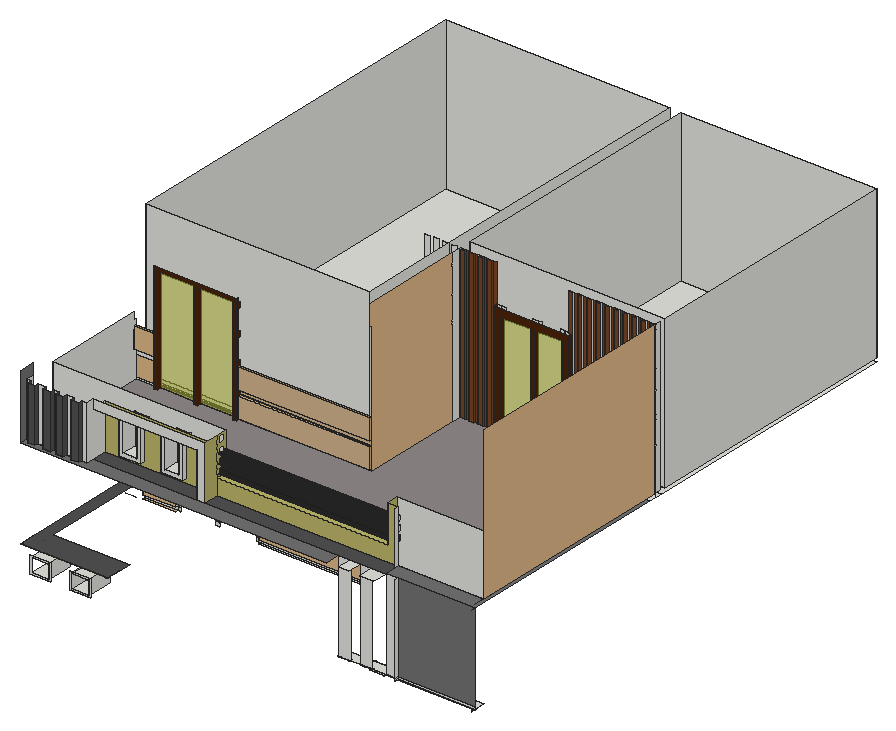
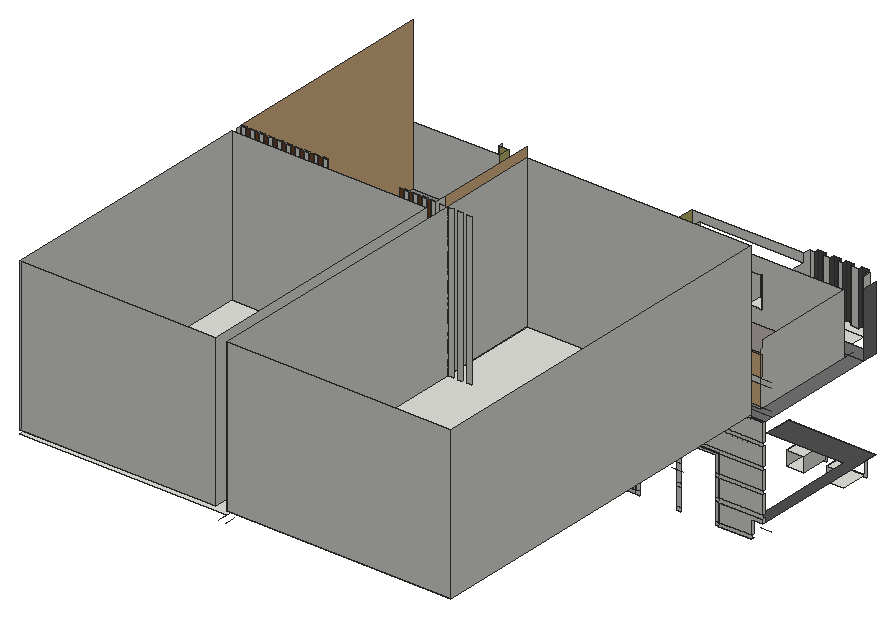
# SketchUp Ruby script. Lengths in inches.
U = 1.inch
M = Sketchup.active_model
def pt(a) = Geom::Point3d.new(a.map { |v| v * U })
def face(e, loops, mat)
  f = e.add_face(loops[0].map { |a| pt(a) })
  loops[1..].each { |l| e.add_face(l.map { |a| pt(a) }).erase! }
  f.material = f.back_material = mat if mat
  f
end
# faces: each face lists its corners as indices into pts; further lists are holes
def faces(e, pts, list, mat = nil) = list.each { |f| face(e, (f[0].is_a?(Array) ? f : [f]).map { |l| l.map { |i| pts[i] } }, mat) }
# xy, xz, yz: faces in a plane at the given z, y or x. An outline is a flat list of corners, or four numbers for a rectangle; further outlines are holes
def ring(l) = l.size == 4 ? [[l[0], l[1]], [l[2], l[1]], [l[2], l[3]], [l[0], l[3]]] : l.each_slice(2).to_a
def flat(e, list, mat, &to3) = list.each { |f| face(e, (f[0].is_a?(Array) ? f : [f]).map { |l| ring(l).map { |u, v| to3.(u, v) } }, mat) }
def xy(e, z, list, mat = nil) = flat(e, list, mat) { |x, y| [x, y, z] }
def xz(e, y, list, mat = nil) = flat(e, list, mat) { |x, z| [x, y, z] }
def yz(e, x, list, mat = nil) = flat(e, list, mat) { |y, z| [x, y, z] }
def lines(e, pts, list) = list.each { |a, b| e.add_line(pt(pts[a]), pt(pts[b])) }
# prism: a flat outline (further loops are holes) pulled along v
def prism(e, loops, v, mat = nil)
  f = face(e, loops, mat); d = Geom::Vector3d.new(v.map { |x| x * U })
  f.pushpull(f.normal.samedirection?(d) ? d.length : -d.length)
end
def box(e, o, s, mat = nil) = prism(e, [[o, [o[0] + s[0], o[1], o[2]], [o[0] + s[0], o[1] + s[1], o[2]], [o[0], o[1] + s[1], o[2]]]], [0, 0, s[2]], mat)
def at(x, y, z, deg = 0) = Geom::Transformation.translation(pt([x, y, z])) * Geom::Transformation.rotation(ORIGIN, Z_AXIS, deg.degrees)
def axes(o, x, y, z) = Geom::Transformation.new([*x, 0, *y, 0, *z, 0, *pt(o).to_a, 1])
def part(name) = M.definitions.add(name)
# library, detail: a bought-in or finely detailed component or shape, given as its bounding box
def library(name, o, s) = part(name).tap { |d| box(d.entities, o, s) }
def detail(e, o, s) = box(e.add_group.entities, o, s)
def put(e, d, t, mat = nil) = e.add_instance(d, t).tap { |i| i.material = mat if mat }
def group(e, t, mat = nil) = e.add_group.tap { |g| g.transformation = t; g.material = mat if mat }.entities
root = M.entities
M.materials.add("[0035_Tan]").color = [210, 180, 140]
M.materials.add("[0036_BurlyWood]").color = [222, 184, 135]
M.materials.add("[0043_SaddleBrown]2").color = [76, 37, 10]
M.materials.add("[0057_DarkKhaki]").color = [189, 183, 107]
M.materials.add("[0135_DarkGray]").color = [81, 81, 81]
M.materials.add("[Blacktop New]").color = [30, 30, 30]
M.materials.add("[Color M05]").color = [114, 114, 114]
M.materials.add("[Stone Marble]").color = [143, 138, 136]
M.materials.add("[Translucent Glass Gray]").color = [209, 214, 54]
M.materials["[Translucent Glass Gray]"].alpha = 0.5
M.materials.add("[Wood Veneer 01]").color = [120, 70, 37]
xy(root,150.27,[[8.88,9,22.59,30],[40.88,9,54.59,30]])
xy(root,154.375,[[8.88,119.875,9,121.875],[100.44,119.875,186.9375,121.875]])
xy(root,154.375,[[9,119.875,34.44,121.875]],"[0036_BurlyWood]")
xy(root,157.3,[[8.88,119.875,34.44,121.875],[100.44,119.875,186.9375,121.875]])
xy(root,161.41,[[8.88,9,22.59,30],[40.88,9,54.59,30]])
xy(root,168,[[269.46,19.25,281.11,19.625],[269.46,19.625,281.11,21],[243.73,21,252.65,22.5625],[281.11,21,290.11,30]])
xy(root,168.11,[[242.89,21,263.86,30],[281.11,21,351,30],[0,119.875,8.88,121.875]])
xy(root,168.11,[[0,9,69.79,9,69.79,30,8.88,30,8.88,119.875,0,119.875]],"[0135_DarkGray]")
xy(root,168.125,[[263.86,21,281.11,30]])
xy(root,171.5,[[100.44,119.875,186.9375,121.875]])
xy(root,171.5,[[0,119.875,9,121.875],[9,119.875,34.44,121.875]],"[0036_BurlyWood]")
xy(root,174.42,[[0,119.875,34.44,121.875],[100.44,119.875,186.9375,121.875]])
xy(root,188.625,[[100.44,119.875,186.9375,121.875]])
xy(root,188.625,[[0,119.875,9,121.875],[9,119.875,34.44,121.875]],"[0036_BurlyWood]")
xy(root,191.55,[[0,119.875,34.44,121.875],[100.44,119.875,186.9375,121.875]])
xy(root,204,[[218.08,193.3125,241.58,196.3125],[244.58,193.3125,266.08,196.3125]])
xy(root,204,[[37.44,118.875,64.75,121.875],[67.75,118.875,97.44,121.875]],"[0043_SaddleBrown]2")
xy(root,205.75,[[0,119.875,9,121.875],[9,119.875,34.44,121.875]])
xy(root,205.75,[[100.44,119.875,186.9375,121.875]],"[0036_BurlyWood]")
xy(root,207,[[34.44,118.875,100.44,121.875]],"[0043_SaddleBrown]2")
xy(root,208.67,[[0,119.875,186.9375,121.875]])
xy(root,210,[[212.08,195.3125,213.9375,196.3125],[216.97,195.3125,222,196.3125],[225.03,195.3125,230.0625,196.3125],[233.09,195.3125,238.125,196.3125],[241.15,195.3125,246.1875,196.3125],
  [249.22,195.3125,254.25,196.3125],[257.28,195.3125,262.3125,196.3125],[265.34,195.3125,270.375,196.3125]])
xy(root,210,[[212.08,193.3125,272.08,193.3125,272.08,196.3125,270.375,196.3125,270.375,195.3125,265.34,195.3125,265.34,196.3125,262.3125,196.3125,262.3125,195.3125,257.28,195.3125,257.28,196.3125,254.25,196.3125,254.25,195.3125,249.22,195.3125,249.22,196.3125,246.1875,196.3125,246.1875,195.3125,241.15,195.3125,241.15,196.3125,238.125,196.3125,238.125,195.3125,233.09,195.3125,233.09,196.3125,230.0625,196.3125,230.0625,195.3125,225.03,195.3125,225.03,196.3125,222,196.3125,222,195.3125,216.97,195.3125,216.97,196.3125,213.9375,196.3125,213.9375,195.3125,212.08,195.3125]],"[0043_SaddleBrown]2")
xy(root,222.875,[[0,119.875,9,121.875],[9,119.875,186.9375,121.875]])
xy(root,225.8,[[0,119.875,186.9375,121.875]])
xy(root,240,[[252.65,9,260.55,21],[269.46,9,281.11,21],[0,119.875,9,121.875],[9,119.875,186.9375,121.875],[345.97,195.3125,345.97,196.3125,186.9375,196.3125,186.9375,207,351,207,351,195.3125],
  [192.78,195.3125,197.8125,196.3125],[200.84,195.3125,205.875,196.3125],[208.9,195.3125,213.9375,196.3125],[216.97,195.3125,222,196.3125],[225.03,195.3125,230.0625,196.3125],
  [233.09,195.3125,238.125,196.3125],[241.15,195.3125,246.1875,196.3125],[249.22,195.3125,254.25,196.3125],[257.28,195.3125,262.3125,196.3125],[265.34,195.3125,270.375,196.3125],
  [273.4,195.3125,278.4375,196.3125],[281.47,195.3125,286.5,196.3125],[289.53,195.3125,294.5625,196.3125],[297.59,195.3125,302.625,196.3125],[305.65,195.3125,310.6875,196.3125],
  [313.72,195.3125,318.75,196.3125],[321.78,195.3125,326.8125,196.3125],[329.84,195.3125,334.875,196.3125],[337.9,195.3125,342.9375,196.3125],[186.9375,196,189.75,196.3125],
  [186.9375,207,351,420]])
xy(root,240,[[0,9,243.73,21],[0,21,0,119.875,186.9375,119.875,186.9375,196,189.75,196,189.75,196.3125,192.78,196.3125,192.78,195.3125,197.8125,195.3125,197.8125,196.3125,200.84,196.3125,200.84,195.3125,205.875,195.3125,205.875,196.3125,208.9,196.3125,208.9,195.3125,213.9375,195.3125,213.9375,196.3125,216.97,196.3125,216.97,195.3125,222,195.3125,222,196.3125,225.03,196.3125,225.03,195.3125,230.0625,195.3125,230.0625,196.3125,233.09,196.3125,233.09,195.3125,238.125,195.3125,238.125,196.3125,241.15,196.3125,241.15,195.3125,246.1875,195.3125,246.1875,196.3125,249.22,196.3125,249.22,195.3125,254.25,195.3125,254.25,196.3125,257.28,196.3125,257.28,195.3125,262.3125,195.3125,262.3125,196.3125,265.34,196.3125,265.34,195.3125,270.375,195.3125,270.375,196.3125,273.4,196.3125,273.4,195.3125,278.4375,195.3125,278.4375,196.3125,281.47,196.3125,281.47,195.3125,286.5,195.3125,286.5,196.3125,289.53,196.3125,289.53,195.3125,294.5625,195.3125,294.5625,196.3125,297.59,196.3125,297.59,195.3125,302.625,195.3125,302.625,196.3125,305.65,196.3125,305.65,195.3125,310.6875,195.3125,310.6875,196.3125,313.72,196.3125,313.72,195.3125,318.75,195.3125,318.75,196.3125,321.78,196.3125,321.78,195.3125,326.8125,195.3125,326.8125,196.3125,329.84,196.3125,329.84,195.3125,334.875,195.3125,334.875,196.3125,337.9,196.3125,337.9,195.3125,342.9375,195.3125,342.9375,196.3125,345.97,196.3125,345.97,195.3125,351,195.3125,351,21]],"[Color M05]")
xy(root,243,[[25.44,109.875,28.44,112.875],[57.44,109.875,60.44,112.875],[88.44,109.875,91.44,112.875],[9,121.875,186.9375,420],[224.67,198,230.67,201],
  [254.61,198,257.61,201],[278.67,198,284.67,201],[196.22,200,200.0625,201],[203.41,200,207.25,201],[210.59,200,214.4375,201],
  [217.78,200,221.625,201],[284.67,200,286.3125,201],[289.66,200,293.5,201],[296.84,200,300.6875,201],[304.03,200,307.875,201],
  [311.22,200,315.0625,201],[318.41,200,322.25,201],[325.59,200,329.4375,201],[332.78,200,336.625,201],[339.97,200,343.8125,201],
  [347.16,200,351,201],[195.9375,210,351,420]])
xy(root,243,[[9,30,351,30,351,200,347.16,200,347.16,201,343.8125,201,343.8125,200,339.97,200,339.97,201,336.625,201,336.625,200,332.78,200,332.78,201,329.4375,201,329.4375,200,325.59,200,325.59,201,322.25,201,322.25,200,318.41,200,318.41,201,315.0625,201,315.0625,200,311.22,200,311.22,201,307.875,201,307.875,200,304.03,200,304.03,201,300.6875,201,300.6875,200,296.84,200,296.84,201,293.5,201,293.5,200,289.66,200,289.66,201,286.3125,201,286.3125,200,284.67,200,284.67,198,278.67,198,278.67,201,257.61,201,257.61,198,254.61,198,254.61,201,230.67,201,230.67,198,224.67,198,224.67,201,221.625,201,221.625,200,217.78,200,217.78,201,214.4375,201,214.4375,200,210.59,200,210.59,201,207.25,201,207.25,200,203.41,200,203.41,201,200.0625,201,200.0625,200,196.22,200,196.22,201,195.9375,201,195.9375,112.875,91.44,112.875,91.44,109.875,88.44,109.875,88.44,112.875,60.44,112.875,60.44,109.875,57.44,109.875,57.44,112.875,28.44,112.875,28.44,109.875,25.44,109.875,25.44,112.875,9,112.875]],"[Stone Marble]")
xy(root,244.47,[[91.44,110.875,195.9375,112.875]],"[0035_Tan]")
xy(root,248.55,[[13.18,0,13.18,3,9.76,3,9.76,9,57.8125,9,57.8125,3,53.28,3,53.28,0,47.49,0,47.49,3,41.34,3,41.34,0,35.56,0,35.56,3,31.22,3,31.22,0,25.43,0,25.43,3,18.97,3,18.97,0],[9.76,9,57.8125,21],[140.4375,9,142.5625,21],[142.5625,9,146.625,21]])
xy(root,248.55,[[57.8125,9,140.4375,21],[146.625,9,290.11,21]],"[0135_DarkGray]")
xy(root,251.61,[[70.9375,18,88.25,21],[104.5625,18,121.875,21]])
xy(root,254.61,[[73.9375,18,85.25,30],[107.5625,18,118.875,30]])
xy(root,260.8125,[[91.44,110.875,195.9375,112.875]],"[0035_Tan]")
xy(root,261.1875,[[146.625,21,282.375,30]],"[0057_DarkKhaki]")
xy(root,264.91,[[91.44,110.875,195.9375,112.875]],"[0035_Tan]")
xy(root,264.91,[[9,110.875,25.44,112.875]],"[0036_BurlyWood]")
xy(root,279.05,[[73.9375,18,85.25,30],[107.5625,18,118.875,30]])
xz(root,0,[[13.18,248.55,18.97,291],[25.43,248.55,31.22,291],[35.56,248.55,41.34,291],[47.49,248.55,53.28,291]],"[0135_DarkGray]")
xz(root,3,[[9.76,248.55,13.18,291],[18.97,248.55,25.43,291],[31.22,248.55,35.56,291],[41.34,248.55,47.49,291],[53.28,248.55,57.8125,291]])
xz(root,9,[[[7.61,149,23.86,162.68],[8.88,150.27,22.59,161.41]],[[39.61,149,55.86,162.68],[40.88,150.27,54.59,161.41]],[0,168,69.79,168.11],[140.4375,248.55,146.625,248.55,146.625,291,57.8125,291,57.8125,284.36,140.4375,284.36]])
xz(root,18,[[[70.9375,251.61,88.25,282.05],[73.9375,254.61,85.25,279.05]],[[104.5625,251.61,121.875,282.05],[107.5625,254.61,118.875,279.05]]])
xz(root,21,[[242.89,168,243.73,168.11],[243.73,168,252.65,168.11],[260.55,168,263.86,168.11],[263.86,168,269.46,168.11],[269.46,168,281.11,168.11],
  [281.11,168,290.11,168.11],[290.11,168,351,168.11],[243.73,168.11,252.65,240],[260.55,168.11,260.55,240,269.46,240,269.46,168.125,263.86,168.125,263.86,168.11],[263.86,168.11,269.46,168.125],
  [269.46,168.11,281.11,168.125],[281.11,168.11,290.11,240],[290.11,168.11,351,169.6875],[140.4375,248.55,142.5625,284.36],[142.5625,248.55,146.625,284.36]])
xz(root,21,[[[57.8125,248.55,140.4375,284.36],[70.9375,251.61,88.25,282.05],[104.5625,251.61,121.875,282.05]],[146.625,248.55,290.11,248.55,290.11,291,282.375,291,282.375,261.1875,146.625,261.1875]],"[0057_DarkKhaki]")
xz(root,21,[[290.11,169.6875,351,240]],"[Color M05]")
xz(root,30,[[263.86,168.11,281.11,168.125],[[9,243,9,291,146.625,291,146.625,261.1875,282.375,261.1875,282.375,291,351,291,351,243],[107.5625,254.61,118.875,279.05],[73.9375,254.61,85.25,279.05]]])
xz(root,109.875,[[25.44,243,28.44,243,28.44,327,57.44,327,57.44,243,60.44,243,60.44,327,88.44,327,88.44,243,91.44,243,91.44,330,25.44,330]],"[0043_SaddleBrown]2")
xz(root,110.875,[[91.44,244.47,195.9375,260.8125],[91.44,264.91,195.9375,281.25]],"[0035_Tan]")
xz(root,110.875,[[9,264.91,25.44,281.25]],"[0036_BurlyWood]")
xz(root,112.875,[[9,243,25.44,244.47],[25.44,243,28.44,244.47],[57.44,243,60.44,244.47],[88.44,243,91.44,244.47],[91.44,243,195.9375,244.47],
  [25.44,244.47,28.44,260.8125],[57.44,244.47,60.44,260.8125],[88.44,244.47,91.44,260.8125],[9,260.8125,25.44,264.91],[25.44,260.8125,28.44,264.91],
  [57.44,260.8125,60.44,264.91],[88.44,260.8125,91.44,264.91],[25.44,264.91,28.44,281.25],[57.44,264.91,60.44,281.25],[88.44,264.91,91.44,281.25]])
xz(root,112.875,[[91.44,244.47,195.9375,260.8125],[91.44,260.8125,195.9375,264.91],[91.44,264.91,195.9375,281.25]],"[0035_Tan]")
xz(root,112.875,[[9,244.47,25.44,260.8125],[9,264.91,25.44,281.25]],"[0036_BurlyWood]")
xz(root,112.875,[[28.44,243,57.44,327],[60.44,243,88.44,327]],"[Translucent Glass Gray]")
xz(root,119.875,[[8.88,157.3,34.44,157.3,34.44,171.5,0,171.5,0,168.11,8.88,168.11],[100.44,157.3,186.9375,171.5],[0,174.42,34.44,188.625],[100.44,174.42,186.9375,188.625],[0,191.55,34.44,205.75],
  [100.44,191.55,186.9375,205.75],[0,208.67,186.9375,222.875],[0,225.8,186.9375,240]],"[0036_BurlyWood]")
xz(root,121.875,[[8.88,154.375,34.44,157.3],[34.44,154.375,37.44,157.3],[64.75,154.375,67.75,157.3],[97.44,154.375,100.44,157.3],[100.44,154.375,186.9375,157.3],
  [8.88,157.3,8.88,168.11,0,168.11,0,171.5,34.44,171.5,34.44,157.3],[34.44,157.3,37.44,171.5],[64.75,157.3,67.75,171.5],[97.44,157.3,100.44,171.5],[100.44,157.3,186.9375,171.5],
  [0,171.5,34.44,174.42],[34.44,171.5,37.44,174.42],[64.75,171.5,67.75,174.42],[97.44,171.5,100.44,174.42],[100.44,171.5,186.9375,174.42],
  [0,174.42,34.44,188.625],[34.44,174.42,37.44,188.625],[64.75,174.42,67.75,188.625],[97.44,174.42,100.44,188.625],[100.44,174.42,186.9375,188.625],
  [0,188.625,34.44,191.55],[34.44,188.625,37.44,191.55],[64.75,188.625,67.75,191.55],[97.44,188.625,100.44,191.55],[100.44,188.625,186.9375,191.55],
  [0,191.55,34.44,205.75],[34.44,191.55,37.44,191.55,37.44,204,64.75,204,64.75,191.55,67.75,191.55,67.75,204,97.44,204,97.44,191.55,100.44,191.55,100.44,205.75,34.44,205.75],[100.44,191.55,186.9375,205.75],[0,205.75,34.44,205.75,34.44,207,100.44,207,100.44,205.75,186.9375,205.75,186.9375,208.67,0,208.67],[34.44,205.75,100.44,207],
  [0,208.67,186.9375,222.875],[0,222.875,186.9375,225.8],[0,225.8,186.9375,240],[9,240,186.9375,243],[9,243,186.9375,363]])
xz(root,195.3125,[[216.97,210,222,240],[225.03,210,230.0625,240],[233.09,210,238.125,240],[241.15,210,246.1875,240],[249.22,210,254.25,240],
  [257.28,210,262.3125,240],[265.34,210,270.375,240]],"[Wood Veneer 01]")
xz(root,196.3125,[[222,204,225.03,210],[225.03,204,230.0625,210],[230.0625,204,233.09,210],[233.09,204,238.125,210],[238.125,204,241.15,210],
  [246.1875,204,249.22,210],[249.22,204,254.25,210],[254.25,204,257.28,210],[257.28,204,262.3125,210],[262.3125,204,265.34,210],
  [216.97,210,222,240],[225.03,210,230.0625,240],[233.09,210,238.125,240],[241.15,210,246.1875,240],[249.22,210,254.25,240],
  [257.28,210,262.3125,240],[265.34,210,270.375,240]])
xz(root,196.3125,[[213.9375,210,216.97,240],[222,210,225.03,240],[230.0625,210,233.09,240],[238.125,210,241.15,240],[246.1875,210,249.22,240],
  [254.25,210,257.28,240],[262.3125,210,265.34,240]],"[Wood Veneer 01]")
xz(root,198,[[224.67,243,230.67,243,230.67,327,254.61,327,254.61,243,257.61,243,257.61,327,278.67,327,278.67,243,284.67,243,284.67,333,224.67,333]],"[0043_SaddleBrown]2")
xz(root,200,[[196.22,243,200.0625,363],[203.41,243,207.25,363],[210.59,243,214.4375,363],[217.78,243,221.625,363],[284.67,243,286.3125,243,286.3125,363,282.47,363,282.47,333,284.67,333],
  [289.66,243,293.5,363],[296.84,243,300.6875,363],[304.03,243,307.875,363],[311.22,243,315.0625,363],[318.41,243,322.25,363],
  [325.59,243,329.4375,363],[332.78,243,336.625,363],[339.97,243,343.8125,363],[347.16,243,351,363]],"[Wood Veneer 01]")
xz(root,201,[[224.67,237,284.67,243],[167.47,243,171.3125,363],[174.66,243,178.5,363],[181.84,243,185.6875,363],[189.03,243,192.875,363],
  [195.9375,243,196.22,363],[196.22,243,200.0625,363],[203.41,243,207.25,363],[210.59,243,214.4375,363],[217.78,243,221.625,363],
  [224.67,243,224.97,333],[224.97,243,228.8125,333],[228.8125,243,228.8125,333,232.16,333,232.16,327,230.67,327,230.67,243],[254.61,243,257.5625,243,257.5625,333,253.72,333,253.72,327,254.61,327],[257.5625,243,257.5625,333,260.91,333,260.91,327,257.61,327,257.61,243],
  [278.67,243,279.125,243,279.125,333,275.28,333,275.28,327,278.67,327],[279.125,243,282.47,333],[282.47,243,284.67,333],[284.67,243,284.67,333,282.47,333,282.47,363,286.3125,363,286.3125,243],[289.66,243,293.5,363],
  [296.84,243,300.6875,363],[304.03,243,307.875,363],[311.22,243,315.0625,363],[318.41,243,322.25,363],[325.59,243,329.4375,363],
  [332.78,243,336.625,363],[339.97,243,343.8125,363],[347.16,243,351,363]])
xz(root,201,[[230.67,243,254.61,327],[257.61,243,278.67,327]],"[Translucent Glass Gray]")
xz(root,201,[[200.0625,243,203.41,363],[207.25,243,210.59,363],[214.4375,243,217.78,363],[221.625,243,224.67,243,224.67,333,224.97,333,224.97,363,221.625,363],[286.3125,243,289.66,363],
  [293.5,243,296.84,363],[300.6875,243,304.03,363],[307.875,243,311.22,363],[315.0625,243,318.41,363],[322.25,243,325.59,363],
  [329.4375,243,332.78,363],[336.625,243,339.97,363],[343.8125,243,347.16,363]],"[Wood Veneer 01]")
xz(root,210,[[195.9375,243,351,363]])
xz(root,420,[[9,243,186.9375,363],[195.9375,243,351,363]])
yz(root,0,[[9,168,21,168.11],[119.875,168.11,121.875,171.5],[119.875,174.42,121.875,188.625],[119.875,191.55,121.875,205.75],[119.875,208.67,121.875,222.875],
  [119.875,225.8,121.875,240]])
yz(root,0,[[9,240,21,291]],"[Color M05]")
yz(root,8.88,[[119.875,157.3,121.875,168.11]])
yz(root,9,[[30,243,112.875,243,112.875,264.91,110.875,264.91,110.875,281.25,112.875,281.25,112.875,285.34,110.875,285.34,110.875,291,30,291],[121.875,243,420,363]])
yz(root,9,[[110.875,264.91,112.875,281.25]],"[0036_BurlyWood]")
yz(root,9.76,[[3,248.55,9,291]])
yz(root,13.18,[[0,248.55,3,291]],"[0135_DarkGray]")
yz(root,18.97,[[0,248.55,3,291]],"[0135_DarkGray]")
yz(root,22.59,[[9,150.27,30,161.41]])
yz(root,25.43,[[0,248.55,3,291]],"[0135_DarkGray]")
yz(root,25.44,[[110.875,264.91,112.875,281.25]],"[0036_BurlyWood]")
yz(root,25.44,[[109.875,243,109.875,330,110.875,330,110.875,326.22,112.875,326.22,112.875,322.125,110.875,322.125,110.875,305.78,112.875,305.78,112.875,301.6875,110.875,301.6875,110.875,285.34,112.875,285.34,112.875,281.25,110.875,281.25,110.875,264.91,112.875,264.91,112.875,243]],"[0043_SaddleBrown]2")
yz(root,28.44,[[109.875,243,112.875,327]],"[0043_SaddleBrown]2")
yz(root,31.22,[[0,248.55,3,291]],"[0135_DarkGray]")
yz(root,34.44,[[119.875,157.3,121.875,171.5],[119.875,174.42,121.875,188.625],[119.875,191.55,121.875,205.75]])
yz(root,35.56,[[0,248.55,3,291]],"[0135_DarkGray]")
yz(root,40.88,[[9,150.27,30,161.41]])
yz(root,41.34,[[0,248.55,3,291]],"[0135_DarkGray]")
yz(root,47.49,[[0,248.55,3,291]],"[0135_DarkGray]")
yz(root,53.28,[[0,248.55,3,291]],"[0135_DarkGray]")
yz(root,54.59,[[9,150.27,30,161.41]])
yz(root,57.44,[[109.875,243,112.875,327]],"[0043_SaddleBrown]2")
yz(root,57.8125,[[3,248.55,21,248.55,21,284.36,9,284.36,9,291,3,291]])
yz(root,60.44,[[109.875,243,112.875,327]],"[0043_SaddleBrown]2")
yz(root,69.79,[[9,168,21,168.11]])
yz(root,70.9375,[[18,251.61,21,282.05]])
yz(root,73.9375,[[18,254.61,30,279.05]])
yz(root,85.25,[[18,254.61,30,279.05]])
yz(root,88.25,[[18,251.61,21,282.05]])
yz(root,88.44,[[109.875,243,112.875,327]],"[0043_SaddleBrown]2")
yz(root,91.44,[[110.875,244.47,112.875,260.8125],[110.875,264.91,112.875,281.25]],"[0035_Tan]")
yz(root,91.44,[[109.875,243,112.875,243,112.875,244.47,110.875,244.47,110.875,260.8125,112.875,260.8125,112.875,264.91,110.875,264.91,110.875,281.25,112.875,281.25,112.875,285.34,110.875,285.34,110.875,301.6875,112.875,301.6875,112.875,305.78,110.875,305.78,110.875,322.125,112.875,322.125,112.875,326.22,110.875,326.22,110.875,330,109.875,330]],"[0043_SaddleBrown]2")
yz(root,100.44,[[119.875,157.3,121.875,171.5],[119.875,174.42,121.875,188.625],[119.875,191.55,121.875,205.75]])
yz(root,104.5625,[[18,251.61,21,282.05]])
yz(root,107.5625,[[18,254.61,30,279.05]])
yz(root,118.875,[[18,254.61,30,279.05]])
yz(root,121.875,[[18,251.61,21,282.05]])
yz(root,140.4375,[[9,248.55,21,284.36]])
yz(root,146.625,[[25.25,251.0625,25.99,251.16,26.68,251.45,27.28,251.9,27.74,252.5,28.02,253.19,28.12,253.9375,28.02,254.68,27.74,255.375,27.28,255.97,26.68,256.43,25.99,256.71,25.25,256.8125,24.5,256.71,23.81,256.43,23.21,255.97,22.76,255.375,22.47,254.68,22.37,253.9375,22.47,253.19,22.76,252.5,23.21,251.9,23.81,251.45,24.5,251.16],[26.72,259.375,27.46,259.47,28.15,259.76,28.75,260.22,29.21,260.8125,29.36,261.1875,24.07,261.1875,24.23,260.8125,24.68,260.22,25.28,259.76,25.97,259.47]])
yz(root,146.625,[[9,248.55,21,291],[[21,261.1875,30,291],[25.25,269,24.5,269.1,23.81,269.39,23.21,269.84,22.76,270.4375,22.47,271.13,22.37,271.875,22.47,272.62,22.76,273.3125,23.21,273.91,23.81,274.37,24.5,274.65,25.25,274.75,25.99,274.65,26.68,274.37,27.28,273.91,27.74,273.3125,28.02,272.62,28.12,271.875,28.02,271.13,27.74,270.4375,27.28,269.84,26.68,269.39,25.99,269.1],[25.25,276,24.5,276.1,23.81,276.39,23.21,276.84,22.76,277.4375,22.47,278.13,22.37,278.875,22.47,279.62,22.76,280.3125,23.21,280.91,23.81,281.37,24.5,281.65,25.25,281.75,25.99,281.65,26.68,281.37,27.28,280.91,27.74,280.3125,28.02,279.62,28.12,278.875,28.02,278.13,27.74,277.4375,27.28,276.84,26.68,276.39,25.99,276.1],[25.25,284.3125,24.5,284.41,23.81,284.7,23.21,285.15,22.76,285.75,22.47,286.44,22.37,287.1875,22.47,287.93,22.76,288.625,23.21,289.22,23.81,289.68,24.5,289.96,25.25,290.0625,25.99,289.96,26.68,289.68,27.28,289.22,27.74,288.625,28.02,287.93,28.12,287.1875,28.02,286.44,27.74,285.75,27.28,285.15,26.68,284.7,25.99,284.41]]],"[0057_DarkKhaki]")
yz(root,186.9375,[[119.875,157.3,121.875,171.5],[119.875,174.42,121.875,188.625],[119.875,191.55,121.875,205.75],[119.875,208.67,121.875,222.875],[119.875,225.8,121.875,240],
  [121.875,240,201,243],[121.875,243,201,363],[201,243,420,363]])
yz(root,195.9375,[[192,243,201,363],[210,243,420,363]])
yz(root,195.9375,[[110.875,244.47,112.875,260.8125],[110.875,264.91,112.875,281.25]],"[0035_Tan]")
yz(root,195.9375,[[112.875,243,192,243,192,363,110.875,363,110.875,346.66,112.875,346.66]],"[0036_BurlyWood]")
yz(root,196.22,[[200,243,201,363]])
yz(root,200.0625,[[200,243,201,363]],"[Wood Veneer 01]")
yz(root,203.41,[[200,243,201,363]])
yz(root,207.25,[[200,243,201,363]],"[Wood Veneer 01]")
yz(root,210.59,[[200,243,201,363]])
yz(root,213.9375,[[195.3125,210,196.3125,240]])
yz(root,214.4375,[[200,243,201,363]],"[Wood Veneer 01]")
yz(root,216.97,[[195.3125,210,196.3125,240]])
yz(root,217.78,[[200,243,201,363]])
yz(root,221.625,[[200,243,201,363]],"[Wood Veneer 01]")
yz(root,222,[[195.3125,210,196.3125,240]])
yz(root,224.67,[[198,243,201,333]],"[0043_SaddleBrown]2")
yz(root,225.03,[[195.3125,210,196.3125,240]])
yz(root,230.0625,[[195.3125,210,196.3125,240]])
yz(root,230.67,[[198,243,201,327]],"[0043_SaddleBrown]2")
yz(root,233.09,[[195.3125,210,196.3125,240]])
yz(root,238.125,[[195.3125,210,196.3125,240]])
yz(root,241.15,[[195.3125,210,196.3125,240]])
yz(root,246.1875,[[195.3125,210,196.3125,240]])
yz(root,249.22,[[195.3125,210,196.3125,240]])
yz(root,254.25,[[195.3125,210,196.3125,240]])
yz(root,254.61,[[198,243,201,327]],"[0043_SaddleBrown]2")
yz(root,257.28,[[195.3125,210,196.3125,240]],"[Wood Veneer 01]")
yz(root,257.61,[[198,243,201,327]],"[0043_SaddleBrown]2")
yz(root,262.3125,[[195.3125,210,196.3125,240]])
yz(root,263.86,[[21,168.11,30,168.125]])
yz(root,265.34,[[195.3125,210,196.3125,240]],"[Wood Veneer 01]")
yz(root,270.375,[[195.3125,210,196.3125,240]])
yz(root,278.67,[[198,243,201,327]],"[0043_SaddleBrown]2")
yz(root,281.11,[[21,168,30,168.11],[21,168.11,30,168.125]])
yz(root,282.375,[[21,261.1875,30,291]],"[0057_DarkKhaki]")
yz(root,284.67,[[200,243,201,333]])
yz(root,284.67,[[198,243,200,333]],"[0043_SaddleBrown]2")
yz(root,286.1875,[[25.25,276,25.99,276.1,26.68,276.39,27.28,276.84,27.74,277.4375,28.02,278.13,28.12,278.875,28.02,279.62,27.74,280.3125,27.28,280.91,26.68,281.37,25.99,281.65,25.25,281.75,24.5,281.65,23.81,281.37,23.21,280.91,22.76,280.3125,22.47,279.62,22.37,278.875,22.47,278.13,22.76,277.4375,23.21,276.84,23.81,276.39,24.5,276.1]])
yz(root,286.3125,[[200,243,201,363]])
yz(root,286.4375,[[25.25,269,25.99,269.1,26.68,269.39,27.28,269.84,27.74,270.4375,28.02,271.13,28.12,271.875,28.02,272.62,27.74,273.3125,27.28,273.91,26.68,274.37,25.99,274.65,25.25,274.75,24.5,274.65,23.81,274.37,23.21,273.91,22.76,273.3125,22.47,272.62,22.37,271.875,22.47,271.13,22.76,270.4375,23.21,269.84,23.81,269.39,24.5,269.1]])
yz(root,289.66,[[200,243,201,363]])
yz(root,290.11,[[18,168,21,168.11],[18,168.11,21,169.6875],[18,169.6875,21,240],[18,248.55,21,291]])
yz(root,293.5,[[200,243,201,363]])
yz(root,296.84,[[200,243,201,363]])
yz(root,300.6875,[[200,243,201,363]])
yz(root,304.03,[[200,243,201,363]])
yz(root,307.875,[[200,243,201,363]])
yz(root,311.22,[[200,243,201,363]],"[Wood Veneer 01]")
yz(root,315.0625,[[200,243,201,363]])
yz(root,318.41,[[200,243,201,363]],"[Wood Veneer 01]")
yz(root,322.25,[[200,243,201,363]])
yz(root,325.59,[[200,243,201,363]],"[Wood Veneer 01]")
yz(root,329.4375,[[200,243,201,363]])
yz(root,332.78,[[200,243,201,363]],"[Wood Veneer 01]")
yz(root,336.625,[[200,243,201,363]])
yz(root,339.97,[[200,243,201,363]],"[Wood Veneer 01]")
yz(root,343.8125,[[200,243,201,363]])
yz(root,347.16,[[200,243,201,363]],"[Wood Veneer 01]")
yz(root,351,[[18,168,21,168.11],[21,168,30,168.11],[200,243,201,363],[201,243,205.5,363],[210,243,420,363]])
yz(root,351,[[30,243,200,363]],"[0036_BurlyWood]")
p = [[146.625,24.5,262.04],[146.625,25.25,261.9375],[286.4375,25.25,261.9375],[286.4375,24.5,262.04],[146.625,25.99,262.04],[286.4375,25.99,262.04],
  [146.625,23.81,262.32],[286.4375,23.81,262.32],[146.625,26.68,262.32],[286.4375,26.68,262.32],[146.625,23.21,262.78],[286.4375,23.21,262.78],
  [146.625,27.28,262.78],[286.4375,27.28,262.78],[146.625,22.76,263.375],[286.4375,22.76,263.375],[146.625,27.74,263.375],[286.4375,27.74,263.375],
  [146.625,22.47,264.07],[286.4375,22.47,264.07],[146.625,28.02,264.07],[286.4375,28.02,264.07],[146.625,22.37,264.8125],[286.4375,22.37,264.8125],
  [146.625,28.12,264.8125],[286.4375,28.12,264.8125],[146.625,22.47,265.56],[286.4375,22.47,265.56],[146.625,28.02,265.56],[286.4375,28.02,265.56],
  [146.625,22.76,266.25],[286.4375,22.76,266.25],[146.625,27.74,266.25],[286.4375,27.74,266.25],[146.625,23.21,266.85],[286.4375,23.21,266.85],
  [146.625,27.28,266.85],[286.4375,27.28,266.85],[146.625,23.81,267.3],[286.4375,23.81,267.3],[146.625,26.68,267.3],[286.4375,26.68,267.3],
  [146.625,24.5,267.59],[286.4375,24.5,267.59],[146.625,25.99,267.59],[286.4375,25.99,267.59],[146.625,25.25,267.6875],[286.4375,25.25,267.6875],
  [146.625,24.5,269.1],[146.625,25.25,269],[286.4375,25.25,269],[286.4375,24.5,269.1],[146.625,25.99,269.1],[286.4375,25.99,269.1],
  [146.625,23.81,269.39],[286.4375,23.81,269.39],[146.625,26.68,269.39],[286.4375,26.68,269.39],[146.625,23.21,269.84],[286.4375,23.21,269.84],
  [146.625,27.28,269.84],[286.4375,27.28,269.84],[146.625,22.76,270.4375],[286.4375,22.76,270.4375],[146.625,27.74,270.4375],[286.4375,27.74,270.4375],
  [146.625,22.47,271.13],[286.4375,22.47,271.13],[146.625,28.02,271.13],[286.4375,28.02,271.13],[146.625,22.37,271.875],[286.4375,22.37,271.875],
  [146.625,28.12,271.875],[286.4375,28.12,271.875],[146.625,22.47,272.62],[286.4375,22.47,272.62],[146.625,28.02,272.62],[286.4375,28.02,272.62],
  [146.625,22.76,273.3125],[286.4375,22.76,273.3125],[146.625,27.74,273.3125],[286.4375,27.74,273.3125],[146.625,23.21,273.91],[286.4375,23.21,273.91],
  [146.625,27.28,273.91],[286.4375,27.28,273.91],[146.625,23.81,274.37],[286.4375,23.81,274.37],[146.625,26.68,274.37],[286.4375,26.68,274.37],
  [146.625,24.5,274.65],[286.4375,24.5,274.65],[146.625,25.99,274.65],[286.4375,25.99,274.65],[146.625,25.25,274.75],[286.4375,25.25,274.75],
  [146.625,24.5,276.1],[146.625,25.25,276],[286.1875,25.25,276],[286.1875,24.5,276.1],[146.625,25.99,276.1],[286.1875,25.99,276.1],
  [146.625,23.81,276.39],[286.1875,23.81,276.39],[146.625,26.68,276.39],[286.1875,26.68,276.39],[146.625,23.21,276.84],[286.1875,23.21,276.84],
  [146.625,27.28,276.84],[286.1875,27.28,276.84],[146.625,22.76,277.4375],[286.1875,22.76,277.4375],[146.625,27.74,277.4375],[286.1875,27.74,277.4375],
  [146.625,22.47,278.13],[286.1875,22.47,278.13],[146.625,28.02,278.13],[286.1875,28.02,278.13],[146.625,22.37,278.875],[286.1875,22.37,278.875],
  [146.625,28.12,278.875],[286.1875,28.12,278.875],[146.625,22.47,279.62],[286.1875,22.47,279.62],[146.625,28.02,279.62],[286.1875,28.02,279.62],
  [351,201,240],[351,201,243],[186.9375,201,240],[180.9375,201,240],[9,201,240],[0,201,240],
  [186.9375,420,240],[186.9375,429,240],[180.9375,420,240],[180.9375,429,240],[351,30,243],[351,21,243],
  [9,30,243],[9,21,243],[91.44,112.875,240],[91.44,112.875,243],[25.44,112.875,243],[25.44,112.875,240.375],
  [9,21,168],[9,21,168.11],[243.73,30,168],[243.73,22.5625,168],[243.52,22.5625,168],[243.52,30,168],
  [243.73,22.5625,168.125],[252.65,22.5625,168],[252.65,22.5625,168.125],[263.86,21,168],[263.86,30,168],[252.65,30,168],
  [9,112.875,264.91],[0,112.875,264.91],[0,112.875,260.8125],[9,112.875,260.8125],[9,112.875,244.47],[0,112.875,244.47],
  [0,112.875,240.375],[0,112.875,240],[9,112.875,240.375],[25.44,112.875,240],[0,112.875,158.625],[9,112.875,158.625],
  [351,21,240],[351,18,240]]
faces(root,p,[[0,1,2,3],[1,4,5,2],[6,0,3,7],[4,8,9,5],[10,6,7,11],[8,12,13,9],[14,10,11,15],[12,16,17,13],
  [18,14,15,19],[16,20,21,17],[22,18,19,23],[20,24,25,21],[26,22,23,27],[24,28,29,25],[30,26,27,31],[28,32,33,29],
  [34,30,31,35],[32,36,37,33],[38,34,35,39],[36,40,41,37],[42,38,39,43],[40,44,45,41],[46,42,43,47],[44,46,47,45],
  [48,49,50,51],[49,52,53,50],[54,48,51,55],[52,56,57,53],[58,54,55,59],[56,60,61,57],[62,58,59,63],[60,64,65,61],
  [66,62,63,67],[64,68,69,65],[70,66,67,71],[68,72,73,69],[74,70,71,75],[72,76,77,73],[78,74,75,79],[76,80,81,77],
  [82,78,79,83],[80,84,85,81],[86,82,83,87],[84,88,89,85],[90,86,87,91],[88,92,93,89],[94,90,91,95],[92,94,95,93],
  [96,97,98,99],[97,100,101,98],[102,96,99,103],[100,104,105,101],[106,102,103,107],[104,108,109,105],[110,106,107,111],[108,112,113,109],
  [114,110,111,115],[112,116,117,113],[118,114,115,119],[116,120,121,117],[122,118,119,123],[120,124,125,121]],"[Blacktop New]")
lines(root,p,[[126,127],[128,129],[130,131],[132,133],[134,135],[136,137],[138,139],[140,141],[142,143],[144,145],[146,147],[148,149],
  [147,150],[151,152],[153,154],[151,155],[156,157],[158,159],[160,161],[162,163],[164,143],[162,164],[143,165],[166,167],
  [168,169]])
